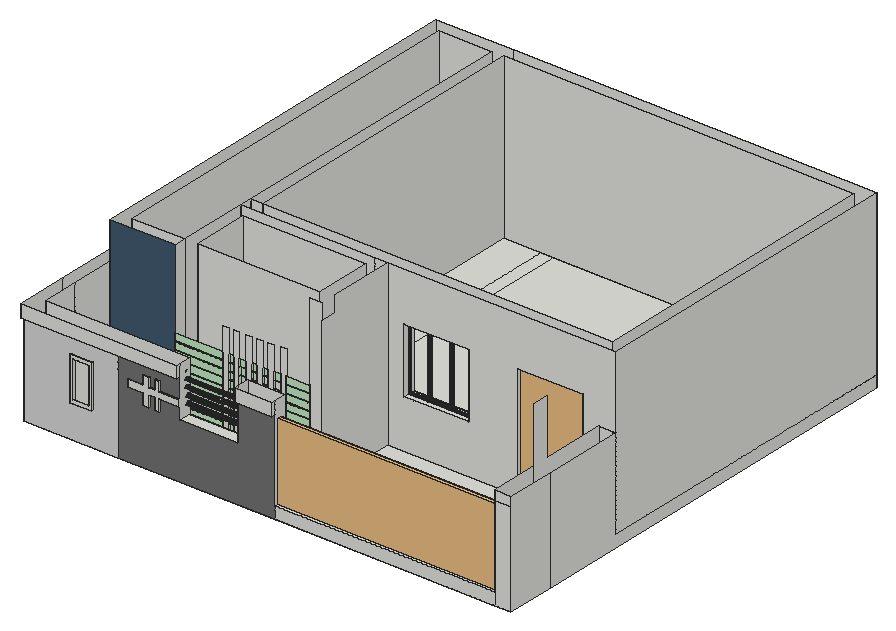
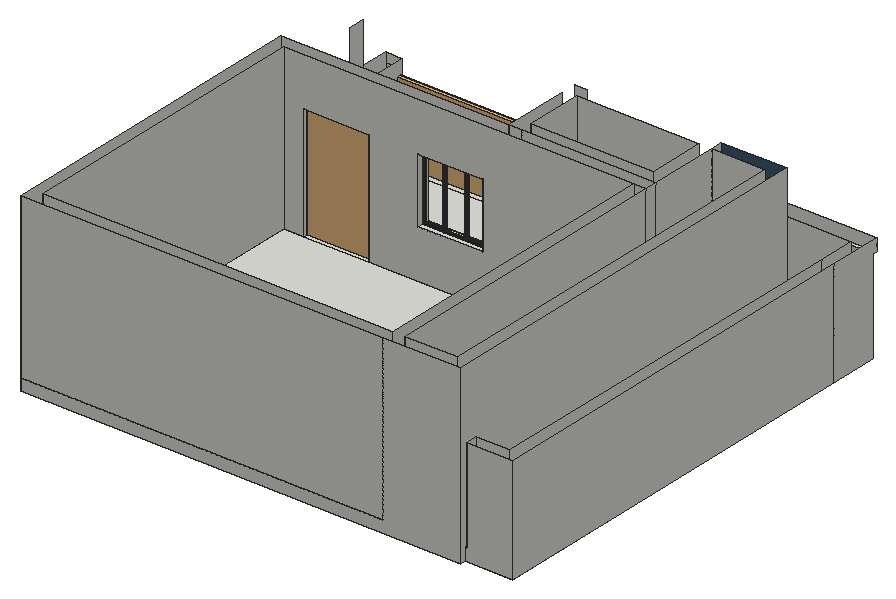
# SketchUp Ruby script. Lengths in inches.
U = 1.inch
M = Sketchup.active_model
def pt(a) = Geom::Point3d.new(a.map { |v| v * U })
def face(e, loops, mat)
  f = e.add_face(loops[0].map { |a| pt(a) })
  loops[1..].each { |l| e.add_face(l.map { |a| pt(a) }).erase! }
  f.material = f.back_material = mat if mat
  f
end
# faces: each face lists its corners as indices into pts; further lists are holes
def faces(e, pts, list, mat = nil) = list.each { |f| face(e, (f[0].is_a?(Array) ? f : [f]).map { |l| l.map { |i| pts[i] } }, mat) }
# xy, xz, yz: faces in a plane at the given z, y or x. An outline is a flat list of corners, or four numbers for a rectangle; further outlines are holes
def ring(l) = l.size == 4 ? [[l[0], l[1]], [l[2], l[1]], [l[2], l[3]], [l[0], l[3]]] : l.each_slice(2).to_a
def flat(e, list, mat, &to3) = list.each { |f| face(e, (f[0].is_a?(Array) ? f : [f]).map { |l| ring(l).map { |u, v| to3.(u, v) } }, mat) }
def xy(e, z, list, mat = nil) = flat(e, list, mat) { |x, y| [x, y, z] }
def xz(e, y, list, mat = nil) = flat(e, list, mat) { |x, z| [x, y, z] }
def yz(e, x, list, mat = nil) = flat(e, list, mat) { |y, z| [x, y, z] }
def lines(e, pts, list) = list.each { |a, b| e.add_line(pt(pts[a]), pt(pts[b])) }
# prism: a flat outline (further loops are holes) pulled along v
def prism(e, loops, v, mat = nil)
  f = face(e, loops, mat); d = Geom::Vector3d.new(v.map { |x| x * U })
  f.pushpull(f.normal.samedirection?(d) ? d.length : -d.length)
end
def box(e, o, s, mat = nil) = prism(e, [[o, [o[0] + s[0], o[1], o[2]], [o[0] + s[0], o[1] + s[1], o[2]], [o[0], o[1] + s[1], o[2]]]], [0, 0, s[2]], mat)
def at(x, y, z, deg = 0) = Geom::Transformation.translation(pt([x, y, z])) * Geom::Transformation.rotation(ORIGIN, Z_AXIS, deg.degrees)
def axes(o, x, y, z) = Geom::Transformation.new([*x, 0, *y, 0, *z, 0, *pt(o).to_a, 1])
def part(name) = M.definitions.add(name)
# library, detail: a bought-in or finely detailed component or shape, given as its bounding box
def library(name, o, s) = part(name).tap { |d| box(d.entities, o, s) }
def detail(e, o, s) = box(e.add_group.entities, o, s)
def put(e, d, t, mat = nil) = e.add_instance(d, t).tap { |i| i.material = mat if mat }
def group(e, t, mat = nil) = e.add_group.tap { |g| g.transformation = t; g.material = mat if mat }.entities
root = M.entities
M.materials.add("Wine2").color = [0, 0, 0]
M.materials["Wine2"].alpha = 0
M.materials.add("[0111_SlateGray]").color = [66, 89, 112]
M.materials.add("[0116_Lavender]").color = [195, 232, 195]
M.materials.add("[0128_White]").color = [214, 214, 214]
M.materials.add("[0130_Gainsboro]").color = [39, 45, 50]
M.materials.add("[0135_DarkGray]").color = [114, 114, 114]
c1 = library("porta 4",[0.2,-5.42,1.33],[46.55,4.72,83.21])
c2 = library("Louvered screen",[0,0,0],[122,4.25,84])
c3 = part("Framed glazing panel")
xy(c3.entities,0,[[0,-0.98,43.07,0],[0,0,43.07,1.4]],"[0130_Gainsboro]")
xy(c3.entities,0.3,[[0.3,-1.43,42.77,-0.98]],"[0130_Gainsboro]")
xy(c3.entities,2.95,[[2.95,-1.43,40.12,-0.63],[2.95,-0.63,40.12,0],[2.95,0,40.12,0.64],[2.95,0.64,40.12,1.4]],"[0130_Gainsboro]")
xy(c3.entities,3.54,[[3.54,-0.63,39.53,0],[3.54,0,39.53,0.64]],"[0130_Gainsboro]")
xy(c3.entities,111.8125,[[3.54,-0.63,39.53,0],[3.54,0,39.53,0.64]],"[0130_Gainsboro]")
xy(c3.entities,112.4,[[2.95,-1.43,40.12,-0.63],[2.95,-0.63,40.12,0],[2.95,0,40.12,0.64],[2.95,0.64,40.12,1.4]],"[0130_Gainsboro]")
xy(c3.entities,115.05,[[0.3,-1.43,42.77,-0.98]],"[0130_Gainsboro]")
xy(c3.entities,115.35,[[0,-0.98,43.07,0],[0,0,43.07,1.4]],"[0130_Gainsboro]")
xz(c3.entities,-1.43,[[[0.3,0.3,42.77,115.05],[2.95,2.95,40.12,112.4]]],"[0130_Gainsboro]")
xz(c3.entities,-0.98,[[[0,0,43.07,115.35],[0.3,0.3,42.77,115.05]]],"[0130_Gainsboro]")
xz(c3.entities,-0.63,[[[2.95,2.95,40.12,112.4],[3.54,3.54,39.53,111.8125]]],"[0130_Gainsboro]")
xz(c3.entities,0,[[3.54,3.54,39.53,111.8125]],"Wine2")
xz(c3.entities,0,[[[0,0,43.07,115.35],[2.95,2.95,40.12,112.4]],[[2.95,2.95,40.12,112.4],[3.54,3.54,39.53,111.8125]]],"[0130_Gainsboro]")
xz(c3.entities,0.64,[[[2.95,2.95,40.12,112.4],[3.54,3.54,39.53,111.8125]]],"[0130_Gainsboro]")
xz(c3.entities,1.4,[[[0,0,43.07,115.35],[2.95,2.95,40.12,112.4]]],"[0130_Gainsboro]")
yz(c3.entities,0,[[-0.98,0,0,115.35],[0,0,1.4,115.35]],"[0130_Gainsboro]")
yz(c3.entities,0.3,[[-1.43,0.3,-0.98,115.05]],"[0130_Gainsboro]")
yz(c3.entities,2.95,[[-1.43,2.95,-0.63,112.4],[-0.63,2.95,0,112.4],[0,2.95,0.64,112.4],[0.64,2.95,1.4,112.4]],"[0130_Gainsboro]")
yz(c3.entities,3.54,[[-0.63,3.54,0,111.8125],[0,3.54,0.64,111.8125]],"[0130_Gainsboro]")
yz(c3.entities,39.53,[[-0.63,3.54,0,111.8125],[0,3.54,0.64,111.8125]],"[0130_Gainsboro]")
yz(c3.entities,40.12,[[-1.43,2.95,-0.63,112.4],[-0.63,2.95,0,112.4],[0,2.95,0.64,112.4],[0.64,2.95,1.4,112.4]],"[0130_Gainsboro]")
yz(c3.entities,42.77,[[-1.43,0.3,-0.98,115.05]],"[0130_Gainsboro]")
yz(c3.entities,43.07,[[-0.98,0,0,115.35],[0,0,1.4,115.35]],"[0130_Gainsboro]")
c4 = part("Glazed window assembly")
put(c4.entities,c3,axes([90.57,1.43,0],[1.05148,0,0],[0,1,0],[0,0,1]))
put(c4.entities,c3,axes([0,1.43,0],[1.05148,0,0],[0,1,0],[0,0,1]))
put(c4.entities,c3,axes([45.29,1.43,0],[1.05148,0,0],[0,1,0],[0,0,1]))
xy(root,-9,[[0,3,359,39],[0,39,0,334.8,35,334.8,35,339,359,339,359,39]])
xy(root,0,[[185.01,3,347,12],[9,12,347,12,347,99,335,99,335,108,287,108,287,99,191,99,191,39,182,39,182,38.5,164.87,38.5,164.87,39,160.62,39,160.62,38.4375,156.37,38.4375,156.37,37.875,152.12,37.875,152.12,38.4375,148.37,38.4375,148.37,37.4375,144.12,37.4375,144.12,38.5,140.12,38.5,140.12,39,135.87,39,135.87,38.375,131.18,38.375,131.18,37.375,126.93,37.375,126.93,38.375,123.62,38.375,123.62,37.5625,119.37,37.5625,119.37,38.5,83,38.5,83,39,9,39],[126.93,37.375,131.18,39],[144.12,37.4375,148.37,39],[119.37,37.5625,123.62,39],
  [152.12,37.875,156.37,39],[123.62,38.375,126.93,39],[131.18,38.375,135.87,39],[148.37,38.4375,152.12,39],[156.37,38.4375,160.62,39],
  [83,38.5,119.37,39],[140.12,38.5,144.12,39],[164.87,38.5,182,39],[9,39,35,39,35,334.8,34,334.8,34,325.8,9,325.8],[[83,39,191,99],[92,48,182,90]],
  [44,48,83,330],[92,48,182,90],[83,99,287,108],[350,99,359,99,359,339,92,339,92,330,350,330],[335,99,350,108],
  [92,108,119,330],[119,108,128,330],[128,108,350,330]])
xy(root,5,[[123.62,38.375,126.93,39],[131.18,38.375,135.87,39],[148.37,38.4375,152.12,39],[156.37,38.4375,160.62,39],[83,38.5,119.37,39],
  [140.12,38.5,144.12,39],[164.87,38.5,182,39]])
xy(root,5.75,[[123.62,38.375,126.93,39],[131.18,38.375,135.87,39],[148.37,38.4375,152.12,39],[156.37,38.4375,160.62,39],[83,38.5,119.37,39],
  [140.12,38.5,144.12,39],[164.87,38.5,182,39]])
xy(root,10.75,[[123.62,38.375,126.93,39],[131.18,38.375,135.87,39],[148.37,38.4375,152.12,39],[156.37,38.4375,160.62,39],[83,38.5,119.37,39],
  [140.12,38.5,144.12,39],[164.87,38.5,182,39]])
xy(root,11.5,[[148.37,38.4375,152.12,39],[156.37,38.4375,160.62,39],[83,38.5,119.37,39],[123.62,38.5,126.93,39],[131.18,38.5,135.87,39],
  [140.12,38.5,144.12,39],[164.87,38.5,182,39]])
xy(root,15.77,[[35.15,2,50.69,3]])
xy(root,16.5,[[148.37,38.4375,152.12,39],[156.37,38.4375,160.62,39],[83,38.5,119.37,39],[123.62,38.5,126.93,39],[131.18,38.5,135.87,39],
  [140.12,38.5,144.12,39],[164.87,38.5,182,39]])
xy(root,17.25,[[148.37,38.4375,152.12,39],[83,38.5,119.37,39],[123.62,38.5,126.93,39],[131.18,38.5,135.87,39],[140.12,38.5,144.12,39],
  [156.37,38.5,160.62,39],[164.87,38.5,182,39]])
xy(root,17.98,[[37.36,2,48.48,3]])
xy(root,22.25,[[148.37,38.4375,152.12,39],[83,38.5,119.37,39],[123.62,38.5,126.93,39],[131.18,38.5,135.87,39],[140.12,38.5,144.12,39],
  [156.37,38.5,160.62,39],[164.87,38.5,182,39]])
xy(root,23,[[83,38.5,119.37,39],[123.62,38.5,126.93,39],[131.18,38.5,135.87,39],[140.12,38.5,144.12,39],[148.37,38.5,152.12,39],
  [156.37,38.5,160.62,39],[164.87,38.5,182,39]])
xy(root,28,[[83,38.5,119.37,39],[123.62,38.5,126.93,39],[131.18,38.5,135.87,39],[140.12,38.5,144.12,39],[148.37,38.5,152.12,39],
  [156.37,38.5,160.62,39],[164.87,38.5,182,39]])
xy(root,28.75,[[135.87,37.4375,140.12,39],[83,38.5,119.37,39],[123.62,38.5,126.93,39],[131.18,38.5,135.87,39],[140.12,38.5,144.12,39],
  [148.37,38.5,152.12,39],[156.37,38.5,160.62,39],[164.87,38.5,182,39]])
xy(root,31.67,[[115.21,3,157.75,12]])
xy(root,32.31,[[97.17,2,100.67,3]])
xy(root,32.63,[[88.58,2,92.7,3]])
xy(root,33.75,[[83,38.5,119.37,39],[123.62,38.5,126.93,39],[131.18,38.5,135.87,39],[140.12,38.5,144.12,39],[148.37,38.5,152.12,39],
  [156.37,38.5,160.62,39],[164.87,38.5,182,39]])
xy(root,34.5,[[83,38.5,119.37,39],[123.62,38.5,126.93,39],[131.18,38.5,135.87,39],[140.12,38.5,144.12,39],[148.37,38.5,152.12,39],
  [156.37,38.5,160.62,39],[164.87,38.5,182,39]])
xy(root,36,[[203,99,251,108]])
xy(root,39.5,[[83,38.5,119.37,39],[123.62,38.5,126.93,39],[131.18,38.5,135.87,39],[140.12,38.5,144.12,39],[148.37,38.5,152.12,39],
  [156.37,38.5,160.62,39],[164.87,38.5,182,39]])
xy(root,40.25,[[155.87,37.875,156.37,38.5],[83,38.5,119.37,39],[123.62,38.5,126.93,39],[131.18,38.5,135.87,39],[140.12,38.5,144.12,39],
  [148.37,38.5,152.12,39],[156.37,38.5,160.62,39],[164.87,38.5,182,39]])
xy(root,40.9,[[77.4,2,88.58,3],[92.7,2,97.17,3],[100.67,2,115.21,3]])
xy(root,45.25,[[155.87,37.875,156.37,38.5],[83,38.5,119.37,39],[123.62,38.5,126.93,39],[131.18,38.5,135.87,39],[140.12,38.5,144.12,39],
  [148.37,38.5,152.12,39],[156.37,38.5,160.62,39],[164.87,38.5,182,39]])
xy(root,45.36,[[37.36,2,48.48,3]])
xy(root,45.83,[[77.4,2,88.58,3],[92.7,2,97.17,3],[100.67,2,115.21,3]])
xy(root,46,[[83,38.5,119.37,39],[131.18,38.5,135.87,39],[140.12,38.5,144.12,39],[148.37,38.5,152.12,39],[156.37,38.5,160.62,39],
  [164.87,38.5,182,39],[123.62,38.625,126.93,39]])
xy(root,47.5625,[[35.15,2,50.69,3]])
xy(root,51,[[83,38.5,119.37,39],[131.18,38.5,135.87,39],[140.12,38.5,144.12,39],[148.37,38.5,152.12,39],[156.37,38.5,160.62,39],
  [164.87,38.5,182,39],[123.62,38.625,126.93,39]])
xy(root,51.75,[[83,38.5,119.37,39],[131.18,38.5,135.87,39],[140.12,38.5,144.12,39],[148.37,38.5,152.12,39],[156.37,38.5,160.62,39],
  [164.87,38.5,182,39],[123.62,38.625,126.93,39]])
xy(root,52.38,[[88.58,2,92.7,3]])
xy(root,52.43,[[97.17,2,100.67,3]])
xy(root,56.75,[[83,38.5,119.37,39],[131.18,38.5,135.87,39],[140.12,38.5,144.12,39],[148.37,38.5,152.12,39],[156.37,38.5,160.62,39],
  [164.87,38.5,182,39],[123.62,38.625,126.93,39]])
xy(root,57.5,[[131.18,38.4375,135.87,39],[83,38.5,119.37,39],[140.12,38.5,144.12,39],[148.37,38.5,152.12,39],[156.37,38.5,160.62,39],
  [164.87,38.5,182,39],[123.62,38.625,126.93,39]])
xy(root,60,[[0,0,115.21,3],[157.75,0,185.01,3]])
xz(root,0,[[0,60,115.21,69],[157.75,60,185.01,69]])
xz(root,2,[[[35.15,15.77,50.69,47.5625],[37.36,17.98,48.48,45.36]],[97.17,32.31,100.67,32.31,100.67,40.9,115.21,40.9,115.21,45.83,100.67,45.83,100.67,52.43,97.17,52.43,97.17,45.83,92.7,45.83,92.7,52.38,88.58,52.38,88.58,45.83,77.4,45.83,77.4,40.9,88.58,40.9,88.58,32.63,92.7,32.63,92.7,40.9,97.17,40.9]])
xz(root,3,[[185.01,-9,347,0],[347,-9,359,60],[37.36,17.98,48.48,45.36],[347,60,359,67]])
xz(root,3,[[[0,-9,69.1875,60],[35.15,15.77,50.69,47.5625]]],"[0128_White]")
xz(root,3,[[69.1875,-9,185.01,-9,185.01,60,157.75,60,157.75,31.67,115.21,31.67,115.21,40.9,100.67,40.9,100.67,32.31,97.17,32.31,97.17,40.9,92.7,40.9,92.7,32.63,88.58,32.63,88.58,40.9,77.4,40.9,77.4,45.83,88.58,45.83,88.58,52.38,92.7,52.38,92.7,45.83,97.17,45.83,97.17,52.43,100.67,52.43,100.67,45.83,115.21,45.83,115.21,60,69.1875,60]],"[0135_DarkGray]")
xz(root,12,[[9,0,9,69,115.21,69,115.21,31.67,157.75,31.67,157.75,69,185.01,69,185.01,0]])
xz(root,37.375,[[126.93,0,131.18,80.25]])
xz(root,37.4375,[[144.12,0,148.37,80.25],[135.87,28.75,140.12,80.25]])
xz(root,37.5625,[[119.37,0,123.62,80.25]])
xz(root,37.875,[[152.12,0,156.37,0,156.37,40.25,155.87,40.25,155.87,45.25,156.37,45.25,156.37,80.25,152.12,80.25]])
xz(root,38.375,[[123.62,0,126.93,5],[131.18,0,135.87,5],[123.62,5.75,126.93,10.75],[131.18,5.75,135.87,10.75]],"[0116_Lavender]")
xz(root,38.4375,[[148.37,0,152.12,5],[156.37,0,160.62,5],[148.37,5.75,152.12,10.75],[156.37,5.75,160.62,10.75],[148.37,11.5,152.12,16.5],
  [156.37,11.5,160.62,16.5],[148.37,17.25,152.12,22.25],[131.18,57.5,135.87,62.5]],"[0116_Lavender]")
xz(root,38.5,[[140.12,0,144.12,5],[155.87,40.25,160.62,45.25],[148.37,46,152.12,51],[156.37,46,160.62,51],[148.37,51.75,152.12,56.75],
  [156.37,51.75,160.62,56.75]])
xz(root,38.5,[[83,0,119.37,5],[164.87,0,182,5],[83,5.75,119.37,10.75],[140.12,5.75,144.12,10.75],[164.87,5.75,182,10.75],
  [83,11.5,119.37,16.5],[123.62,11.5,126.93,16.5],[131.18,11.5,135.87,16.5],[140.12,11.5,144.12,16.5],[164.87,11.5,182,16.5],
  [83,17.25,119.37,22.25],[123.62,17.25,126.93,22.25],[131.18,17.25,135.87,22.25],[140.12,17.25,144.12,22.25],[156.37,17.25,160.62,22.25],
  [164.87,17.25,182,22.25],[83,23,119.37,28],[123.62,23,126.93,28],[131.18,23,135.87,28],[140.12,23,144.12,28],
  [148.37,23,152.12,28],[156.37,23,160.62,28],[164.87,23,182,28],[83,28.75,119.37,33.75],[123.62,28.75,126.93,33.75],
  [131.18,28.75,135.87,33.75],[140.12,28.75,144.12,33.75],[148.37,28.75,152.12,33.75],[156.37,28.75,160.62,33.75],[164.87,28.75,182,33.75],
  [83,34.5,119.37,39.5],[123.62,34.5,126.93,39.5],[131.18,34.5,135.87,39.5],[140.12,34.5,144.12,39.5],[148.37,34.5,152.12,39.5],
  [156.37,34.5,160.62,39.5],[164.87,34.5,182,39.5],[83,40.25,119.37,45.25],[123.62,40.25,126.93,45.25],[131.18,40.25,135.87,45.25],
  [140.12,40.25,144.12,45.25],[148.37,40.25,152.12,45.25],[164.87,40.25,182,45.25],[83,46,119.37,51],[131.18,46,135.87,51],
  [140.12,46,144.12,51],[164.87,46,182,51],[83,51.75,119.37,56.75],[131.18,51.75,135.87,56.75],[140.12,51.75,144.12,56.75],
  [164.87,51.75,182,56.75],[83,57.5,119.37,62.5],[140.12,57.5,144.12,62.5],[148.37,57.5,152.12,62.5],[156.37,57.5,160.62,62.5],
  [164.87,57.5,182,62.5]],"[0116_Lavender]")
xz(root,38.625,[[123.62,46,126.93,51],[123.62,51.75,126.93,56.75],[123.62,57.5,126.93,62.5]],"[0116_Lavender]")
xz(root,39,[[135.87,0,140.12,28.75],[160.62,0,164.87,28],[182,0,191,120],[83,5,119.37,5.75],[123.62,5,126.93,5.75],
  [131.18,5,135.87,5.75],[140.12,5,144.12,5.75],[148.37,5,152.12,5.75],[156.37,5,160.62,5.75],[164.87,5,182,5.75],
  [83,10.75,119.37,11.5],[123.62,10.75,126.93,11.5],[131.18,10.75,135.87,11.5],[140.12,10.75,144.12,11.5],[148.37,10.75,152.12,11.5],
  [156.37,10.75,160.62,11.5],[164.87,10.75,182,11.5],[83,16.5,119.37,17.25],[123.62,16.5,126.93,17.25],[131.18,16.5,135.87,17.25],
  [140.12,16.5,144.12,17.25],[148.37,16.5,152.12,17.25],[156.37,16.5,160.62,17.25],[164.87,16.5,182,17.25],[83,22.25,119.37,23],
  [123.62,22.25,126.93,23],[131.18,22.25,135.87,23],[140.12,22.25,144.12,23],[148.37,22.25,152.12,23],[156.37,22.25,160.62,23],
  [164.87,22.25,182,23],[83,28,119.37,28.75],[123.62,28,126.93,28.75],[131.18,28,135.87,28.75],[140.12,28,144.12,28.75],
  [148.37,28,152.12,28.75],[156.37,28,160.62,28.75],[160.62,28,164.87,80.25],[164.87,28,182,28.75],[83,33.75,119.37,34.5],
  [123.62,33.75,126.93,34.5],[131.18,33.75,135.87,34.5],[140.12,33.75,144.12,34.5],[148.37,33.75,152.12,34.5],[156.37,33.75,160.62,34.5],
  [164.87,33.75,182,34.5],[83,39.5,119.37,40.25],[123.62,39.5,126.93,40.25],[131.18,39.5,135.87,40.25],[140.12,39.5,144.12,40.25],
  [148.37,39.5,152.12,40.25],[156.37,39.5,160.62,40.25],[164.87,39.5,182,40.25],[83,45.25,119.37,46],[123.62,45.25,126.93,46],
  [131.18,45.25,135.87,46],[140.12,45.25,144.12,46],[148.37,45.25,152.12,46],[156.37,45.25,160.62,46],[164.87,45.25,182,46],
  [83,51,119.37,51.75],[123.62,51,126.93,51.75],[131.18,51,135.87,51.75],[140.12,51,144.12,51.75],[148.37,51,152.12,51.75],
  [156.37,51,160.62,51.75],[164.87,51,182,51.75],[83,56.75,119.37,57.5],[123.62,56.75,126.93,57.5],[131.18,56.75,135.87,57.5],
  [140.12,56.75,144.12,57.5],[148.37,56.75,152.12,57.5],[156.37,56.75,160.62,57.5],[164.87,56.75,182,57.5]])
xz(root,39,[[35,0,83,120]],"[0111_SlateGray]")
xz(root,48,[[44,0,83,120],[92,0,182,120]])
xz(root,90,[[92,0,182,120]])
xz(root,99,[[83,0,182,120],[182,0,191,120],[[191,0,287,0,287,84,335,84,335,0,347,0,347,67,359,67,359,120,191,120],[203,36,251,84]]])
xz(root,108,[[83,0,92,120],[[92,0,92,120,350,120,350,0,335,0,335,84,287,84,287,0],[203,36,251,84]]])
xz(root,325.8,[[9,0,34,69]])
xz(root,330,[[44,0,83,120],[92,0,350,120]])
xz(root,334.8,[[0,-9,0,69,34,69,34,0,35,0,35,-9]])
xz(root,339,[[35,-9,35,120,92,120,92,0,359,0,359,-9],[92,0,359,120]])
yz(root,0,[[3,-9,3,60,0,60,0,69,39,69,39,-9],[39,-9,334.8,69]])
yz(root,9,[[12,0,39,69],[39,0,325.8,69]])
yz(root,34,[[325.8,0,334.8,69]])
yz(root,35,[[334.8,-9,334.8,0,39,0,39,120,339,120,339,-9]])
yz(root,35.15,[[2,15.77,3,47.5625]])
yz(root,37.36,[[2,17.98,3,45.36]])
yz(root,44,[[48,0,330,120]])
yz(root,48.48,[[2,17.98,3,45.36]])
yz(root,50.69,[[2,15.77,3,47.5625]])
yz(root,77.4,[[2,40.9,3,45.83]])
yz(root,83,[[38.5,0,39,5],[39,0,48,120],[48,0,99,120],[99,0,108,120],[108,0,330,120],
  [38.5,5.75,39,10.75],[38.5,11.5,39,16.5],[38.5,17.25,39,22.25],[38.5,23,39,28],[38.5,28.75,39,33.75],
  [38.5,34.5,39,39.5],[38.5,40.25,39,45.25],[38.5,46,39,51],[38.5,51.75,39,56.75],[38.5,57.5,39,62.5]])
yz(root,88.58,[[2,32.63,3,40.9],[2,45.83,3,52.38]])
yz(root,92,[[48,0,90,120],[108,0,330,120]])
yz(root,92.7,[[2,32.63,3,40.9],[2,45.83,3,52.38]])
yz(root,97.17,[[2,32.31,3,40.9],[2,45.83,3,52.43]])
yz(root,100.67,[[2,32.31,3,40.9],[2,45.83,3,52.43]])
yz(root,115.21,[[[3,31.67,12,31.67,12,69,3,69,3,45.83,2,45.83,2,40.9,3,40.9],[9.375,44.125,9.05,44.17,8.75,44.29,8.49,44.49,8.29,44.75,8.17,45.05,8.125,45.375,8.17,45.7,8.29,46,8.49,46.26,8.75,46.46,9.05,46.58,9.375,46.625,9.7,46.58,10,46.46,10.26,46.26,10.46,46,10.58,45.7,10.625,45.375,10.58,45.05,10.46,44.75,10.26,44.49,10,44.29,9.7,44.17],[9.375,38.875,9.05,38.92,8.75,39.04,8.49,39.24,8.29,39.5,8.17,39.8,8.125,40.125,8.17,40.45,8.29,40.75,8.49,41.01,8.75,41.21,9.05,41.33,9.375,41.375,9.7,41.33,10,41.21,10.26,41.01,10.46,40.75,10.58,40.45,10.625,40.125,10.58,39.8,10.46,39.5,10.26,39.24,10,39.04,9.7,38.92],[8.625,50.42,8.33,50.46,8.0625,50.57,7.83,50.75,7.65,50.99,7.54,51.26,7.5,51.55,7.54,51.84,7.65,52.11,7.83,52.34,8.0625,52.52,8.33,52.63,8.625,52.67,8.92,52.63,9.1875,52.52,9.42,52.34,9.6,52.11,9.71,51.84,9.75,51.55,9.71,51.26,9.6,50.99,9.42,50.75,9.1875,50.57,8.92,50.46],[8.625,60.67,8.33,60.71,8.0625,60.82,7.83,61,7.65,61.24,7.54,61.51,7.5,61.8,7.54,62.09,7.65,62.36,7.83,62.59,8.0625,62.77,8.33,62.88,8.625,62.92,8.92,62.88,9.1875,62.77,9.42,62.59,9.6,62.36,9.71,62.09,9.75,61.8,9.71,61.51,9.6,61.24,9.42,61,9.1875,60.82,8.92,60.71],[8.625,55.8,8.33,55.84,8.0625,55.95,7.83,56.13,7.65,56.36,7.54,56.63,7.5,56.92,7.54,57.21,7.65,57.49,7.83,57.72,8.0625,57.9,8.33,58.01,8.625,58.05,8.92,58.01,9.1875,57.9,9.42,57.72,9.6,57.49,9.71,57.21,9.75,56.92,9.71,56.63,9.6,56.36,9.42,56.13,9.1875,55.95,8.92,55.84]],[0,60,3,69]])
yz(root,119.37,[[37.5625,0,38.5,5],[37.5625,5,39,5.75],[37.5625,5.75,38.5,10.75],[37.5625,10.75,39,11.5],[37.5625,11.5,38.5,16.5],
  [37.5625,16.5,39,17.25],[37.5625,17.25,38.5,22.25],[37.5625,22.25,39,23],[37.5625,23,38.5,28],[37.5625,28,39,28.75],
  [37.5625,28.75,38.5,33.75],[37.5625,33.75,39,34.5],[37.5625,34.5,38.5,39.5],[37.5625,39.5,39,40.25],[37.5625,40.25,38.5,45.25],
  [37.5625,45.25,39,46],[37.5625,46,38.5,51],[37.5625,51,39,51.75],[37.5625,51.75,38.5,56.75],[37.5625,56.75,39,57.5],
  [37.5625,57.5,38.5,62.5]])
yz(root,123.62,[[37.5625,0,38.375,5],[37.5625,5,39,5.75],[37.5625,5.75,38.375,10.75],[37.5625,10.75,39,11.5],[37.5625,11.5,38.5,16.5],
  [37.5625,16.5,39,17.25],[37.5625,17.25,38.5,22.25],[37.5625,22.25,39,23],[37.5625,23,38.5,28],[37.5625,28,39,28.75],
  [37.5625,28.75,38.5,33.75],[37.5625,33.75,39,34.5],[37.5625,34.5,38.5,39.5],[37.5625,39.5,39,40.25],[37.5625,40.25,38.5,45.25],
  [37.5625,45.25,39,46],[37.5625,46,38.625,51],[37.5625,51,39,51.75],[37.5625,51.75,38.625,56.75],[37.5625,56.75,39,57.5],
  [37.5625,57.5,38.625,62.5]])
yz(root,126.93,[[37.375,0,38.375,5],[37.375,5,39,5.75],[37.375,5.75,38.375,10.75],[37.375,10.75,39,11.5],[37.375,11.5,38.5,16.5],
  [37.375,16.5,39,17.25],[37.375,17.25,38.5,22.25],[37.375,22.25,39,23],[37.375,23,38.5,28],[37.375,28,39,28.75],
  [37.375,28.75,38.5,33.75],[37.375,33.75,39,34.5],[37.375,34.5,38.5,39.5],[37.375,39.5,39,40.25],[37.375,40.25,38.5,45.25],
  [37.375,45.25,39,46],[37.375,46,38.625,51],[37.375,51,39,51.75],[37.375,51.75,38.625,56.75],[37.375,56.75,39,57.5],
  [37.375,57.5,38.625,62.5]])
yz(root,131.18,[[37.375,0,38.375,5],[37.375,5,39,5.75],[37.375,5.75,38.375,10.75],[37.375,10.75,39,11.5],[37.375,11.5,38.5,16.5],
  [37.375,16.5,39,17.25],[37.375,17.25,38.5,22.25],[37.375,22.25,39,23],[37.375,23,38.5,28],[37.375,28,39,28.75],
  [37.375,28.75,38.5,33.75],[37.375,33.75,39,34.5],[37.375,34.5,38.5,39.5],[37.375,39.5,39,40.25],[37.375,40.25,38.5,45.25],
  [37.375,45.25,39,46],[37.375,46,38.5,51],[37.375,51,39,51.75],[37.375,51.75,38.5,56.75],[37.375,56.75,39,57.5],
  [37.375,57.5,38.4375,62.5]])
yz(root,135.87,[[38.375,0,39,5],[38.375,5.75,39,10.75],[38.5,11.5,39,16.5],[38.5,17.25,39,22.25],[38.5,23,39,28],
  [37.4375,28.75,38.5,33.75],[37.4375,33.75,39,34.5],[37.4375,34.5,38.5,39.5],[37.4375,39.5,39,40.25],[37.4375,40.25,38.5,45.25],
  [37.4375,45.25,39,46],[37.4375,46,38.5,51],[37.4375,51,39,51.75],[37.4375,51.75,38.5,56.75],[37.4375,56.75,39,57.5],
  [37.4375,57.5,38.4375,62.5]])
yz(root,140.12,[[38.5,0,39,5],[38.5,5.75,39,10.75],[38.5,11.5,39,16.5],[38.5,17.25,39,22.25],[38.5,23,39,28],
  [37.4375,28.75,38.5,33.75],[37.4375,33.75,39,34.5],[37.4375,34.5,38.5,39.5],[37.4375,39.5,39,40.25],[37.4375,40.25,38.5,45.25],
  [37.4375,45.25,39,46],[37.4375,46,38.5,51],[37.4375,51,39,51.75],[37.4375,51.75,38.5,56.75],[37.4375,56.75,39,57.5],
  [37.4375,57.5,38.5,62.5]])
yz(root,144.12,[[37.4375,0,38.5,5],[37.4375,5,39,5.75],[37.4375,5.75,38.5,10.75],[37.4375,10.75,39,11.5],[37.4375,11.5,38.5,16.5],
  [37.4375,16.5,39,17.25],[37.4375,17.25,38.5,22.25],[37.4375,22.25,39,23],[37.4375,23,38.5,28],[37.4375,28,39,28.75],
  [37.4375,28.75,38.5,33.75],[37.4375,33.75,39,34.5],[37.4375,34.5,38.5,39.5],[37.4375,39.5,39,40.25],[37.4375,40.25,38.5,45.25],
  [37.4375,45.25,39,46],[37.4375,46,38.5,51],[37.4375,51,39,51.75],[37.4375,51.75,38.5,56.75],[37.4375,56.75,39,57.5],
  [37.4375,57.5,38.5,62.5]])
yz(root,148.37,[[37.4375,0,38.4375,5],[37.4375,5,39,5.75],[37.4375,5.75,38.4375,10.75],[37.4375,10.75,39,11.5],[37.4375,11.5,38.4375,16.5],
  [37.4375,16.5,39,17.25],[37.4375,17.25,38.4375,22.25],[37.4375,22.25,39,23],[37.4375,23,38.5,28],[37.4375,28,39,28.75],
  [37.4375,28.75,38.5,33.75],[37.4375,33.75,39,34.5],[37.4375,34.5,38.5,39.5],[37.4375,39.5,39,40.25],[37.4375,40.25,38.5,45.25],
  [37.4375,45.25,39,46],[37.4375,46,38.5,51],[37.4375,51,39,51.75],[37.4375,51.75,38.5,56.75],[37.4375,56.75,39,57.5],
  [37.4375,57.5,38.5,62.5]])
yz(root,152.12,[[37.875,0,38.4375,5],[37.875,5,39,5.75],[37.875,5.75,38.4375,10.75],[37.875,10.75,39,11.5],[37.875,11.5,38.4375,16.5],
  [37.875,16.5,39,17.25],[37.875,17.25,38.4375,22.25],[37.875,22.25,39,23],[37.875,23,38.5,28],[37.875,28,39,28.75],
  [37.875,28.75,38.5,33.75],[37.875,33.75,39,34.5],[37.875,34.5,38.5,39.5],[37.875,39.5,39,40.25],[37.875,40.25,38.5,45.25],
  [37.875,45.25,39,46],[37.875,46,38.5,51],[37.875,51,39,51.75],[37.875,51.75,38.5,56.75],[37.875,56.75,39,57.5],
  [37.875,57.5,38.5,62.5]])
yz(root,155.87,[[37.875,40.25,38.5,45.25]])
yz(root,156.37,[[37.875,0,38.4375,5],[37.875,5,39,5.75],[37.875,5.75,38.4375,10.75],[37.875,10.75,39,11.5],[37.875,11.5,38.4375,16.5],
  [37.875,16.5,39,17.25],[37.875,17.25,38.5,22.25],[37.875,22.25,39,23],[37.875,23,38.5,28],[37.875,28,39,28.75],
  [37.875,28.75,38.5,33.75],[37.875,33.75,39,34.5],[37.875,34.5,38.5,39.5],[37.875,39.5,39,40.25],[37.875,45.25,39,46],
  [37.875,46,38.5,51],[37.875,51,39,51.75],[37.875,51.75,38.5,56.75],[37.875,56.75,39,57.5],[37.875,57.5,38.5,62.5]])
yz(root,157.59,[[9.375,38.875,9.7,38.92,10,39.04,10.26,39.24,10.46,39.5,10.58,39.8,10.625,40.125,10.58,40.45,10.46,40.75,10.26,41.01,10,41.21,9.7,41.33,9.375,41.375,9.05,41.33,8.75,41.21,8.49,41.01,8.29,40.75,8.17,40.45,8.125,40.125,8.17,39.8,8.29,39.5,8.49,39.24,8.75,39.04,9.05,38.92]])
yz(root,157.75,[[[3,31.67,12,69],[9.375,44.125,9.7,44.17,10,44.29,10.26,44.49,10.46,44.75,10.58,45.05,10.625,45.375,10.58,45.7,10.46,46,10.26,46.26,10,46.46,9.7,46.58,9.375,46.625,9.05,46.58,8.75,46.46,8.49,46.26,8.29,46,8.17,45.7,8.125,45.375,8.17,45.05,8.29,44.75,8.49,44.49,8.75,44.29,9.05,44.17],[8.625,50.42,8.92,50.46,9.1875,50.57,9.42,50.75,9.6,50.99,9.71,51.26,9.75,51.55,9.71,51.84,9.6,52.11,9.42,52.34,9.1875,52.52,8.92,52.63,8.625,52.67,8.33,52.63,8.0625,52.52,7.83,52.34,7.65,52.11,7.54,51.84,7.5,51.55,7.54,51.26,7.65,50.99,7.83,50.75,8.0625,50.57,8.33,50.46]],[0,60,3,69]])
yz(root,157.9,[[8.625,55.8,8.92,55.84,9.1875,55.95,9.42,56.13,9.6,56.36,9.71,56.63,9.75,56.92,9.71,57.21,9.6,57.49,9.42,57.72,9.1875,57.9,8.92,58.01,8.625,58.05,8.33,58.01,8.0625,57.9,7.83,57.72,7.65,57.49,7.54,57.21,7.5,56.92,7.54,56.63,7.65,56.36,7.83,56.13,8.0625,55.95,8.33,55.84]])
yz(root,160.62,[[38.4375,0,39,5],[38.4375,5.75,39,10.75],[38.4375,11.5,39,16.5],[38.5,17.25,39,22.25],[38.5,23,39,28],
  [38.5,28.75,39,33.75],[38.5,34.5,39,39.5],[38.5,40.25,39,45.25],[38.5,46,39,51],[38.5,51.75,39,56.75],
  [38.5,57.5,39,62.5]])
yz(root,164.87,[[38.5,0,39,5],[38.5,5.75,39,10.75],[38.5,11.5,39,16.5],[38.5,17.25,39,22.25],[38.5,23,39,28],
  [38.5,28.75,39,33.75],[38.5,34.5,39,39.5],[38.5,40.25,39,45.25],[38.5,46,39,51],[38.5,51.75,39,56.75],
  [38.5,57.5,39,62.5]])
yz(root,182,[[38.5,0,39,5],[48,0,90,120],[38.5,5.75,39,10.75],[38.5,11.5,39,16.5],[38.5,17.25,39,22.25],
  [38.5,23,39,28],[38.5,28.75,39,33.75],[38.5,34.5,39,39.5],[38.5,40.25,39,45.25],[38.5,46,39,51],
  [38.5,51.75,39,56.75],[38.5,57.5,39,62.5]])
yz(root,185.01,[[3,0,12,69],[0,60,3,69]])
yz(root,191,[[39,0,99,0,99,120,51,120,51,108,39,108]])
yz(root,203,[[99,36,108,84]])
yz(root,251,[[99,36,108,84]])
yz(root,287,[[99,0,108,84]])
yz(root,335,[[99,0,108,84]])
yz(root,347,[[3,0,39,67],[39,0,39,108,51,108,51,67,99,67,99,0]])
yz(root,350,[[108,0,330,120]])
yz(root,359,[[3,-9,39,67],[39,-9,339,-9,339,0,99,0,99,67,39,67],[99,0,339,120]])
p = [[115.21,8.75,39.04],[115.21,9.05,38.92],[157.59,9.05,38.92],[157.59,8.75,39.04],[115.21,9.375,38.875],[157.59,9.375,38.875],
  [115.21,9.7,38.92],[157.59,9.7,38.92],[115.21,10,39.04],[157.59,10,39.04],[115.21,8.49,39.24],[157.59,8.49,39.24],
  [115.21,10.26,39.24],[157.59,10.26,39.24],[115.21,8.29,39.5],[157.59,8.29,39.5],[115.21,10.46,39.5],[157.59,10.46,39.5],
  [115.21,8.17,39.8],[157.59,8.17,39.8],[115.21,10.58,39.8],[157.59,10.58,39.8],[115.21,8.125,40.125],[157.59,8.125,40.125],
  [115.21,10.625,40.125],[157.59,10.625,40.125],[115.21,8.17,40.45],[157.59,8.17,40.45],[115.21,10.58,40.45],[157.59,10.58,40.45],
  [115.21,8.29,40.75],[157.59,8.29,40.75],[115.21,10.46,40.75],[157.59,10.46,40.75],[115.21,8.49,41.01],[157.59,8.49,41.01],
  [115.21,10.26,41.01],[157.59,10.26,41.01],[115.21,8.75,41.21],[157.59,8.75,41.21],[115.21,10,41.21],[157.59,10,41.21],
  [115.21,9.05,41.33],[157.59,9.05,41.33],[115.21,9.7,41.33],[157.59,9.7,41.33],[115.21,9.375,41.375],[157.59,9.375,41.375],
  [115.21,9.05,44.17],[115.21,9.375,44.125],[157.75,9.375,44.125],[157.75,9.05,44.17],[115.21,9.7,44.17],[157.75,9.7,44.17],
  [115.21,8.75,44.29],[157.75,8.75,44.29],[115.21,10,44.29],[157.75,10,44.29],[115.21,8.49,44.49],[157.75,8.49,44.49],
  [115.21,10.26,44.49],[157.75,10.26,44.49],[115.21,8.29,44.75],[157.75,8.29,44.75],[115.21,10.46,44.75],[157.75,10.46,44.75],
  [115.21,8.17,45.05],[157.75,8.17,45.05],[115.21,10.58,45.05],[157.75,10.58,45.05],[115.21,8.125,45.375],[157.75,8.125,45.375],
  [115.21,10.625,45.375],[157.75,10.625,45.375],[115.21,8.17,45.7],[157.75,8.17,45.7],[115.21,10.58,45.7],[157.75,10.58,45.7],
  [115.21,8.29,46],[157.75,8.29,46],[115.21,10.46,46],[157.75,10.46,46],[115.21,8.49,46.26],[157.75,8.49,46.26],
  [115.21,10.26,46.26],[157.75,10.26,46.26],[115.21,8.75,46.46],[157.75,8.75,46.46],[115.21,10,46.46],[157.75,10,46.46],
  [115.21,9.05,46.58],[157.75,9.05,46.58],[115.21,9.7,46.58],[157.75,9.7,46.58],[115.21,9.375,46.625],[157.75,9.375,46.625],
  [115.21,8.33,50.46],[115.21,8.625,50.42],[157.75,8.625,50.42],[157.75,8.33,50.46],[115.21,8.92,50.46],[157.75,8.92,50.46],
  [115.21,8.0625,50.57],[157.75,8.0625,50.57],[115.21,9.1875,50.57],[157.75,9.1875,50.57],[115.21,7.83,50.75],[157.75,7.83,50.75],
  [115.21,9.42,50.75],[157.75,9.42,50.75],[115.21,7.65,50.99],[157.75,7.65,50.99],[115.21,9.6,50.99],[157.75,9.6,50.99],
  [115.21,7.54,51.26],[157.75,7.54,51.26],[115.21,9.71,51.26],[157.75,9.71,51.26],[115.21,7.5,51.55],[157.75,7.5,51.55],
  [115.21,9.75,51.55],[157.75,9.75,51.55],[115.21,7.54,51.84],[157.75,7.54,51.84],[115.21,9.71,51.84],[157.75,9.71,51.84],
  [115.21,7.65,52.11],[157.75,7.65,52.11],[115.21,9.6,52.11],[157.75,9.6,52.11],[115.21,7.83,52.34],[157.75,7.83,52.34],
  [115.21,9.42,52.34],[157.75,9.42,52.34],[115.21,8.0625,52.52],[157.75,8.0625,52.52],[115.21,9.1875,52.52],[157.75,9.1875,52.52],
  [115.21,8.33,52.63],[157.75,8.33,52.63],[115.21,8.92,52.63],[157.75,8.92,52.63],[115.21,8.625,52.67],[157.75,8.625,52.67],
  [115.21,8.0625,55.95],[115.21,8.33,55.84],[157.9,8.33,55.84],[157.9,8.0625,55.95],[115.21,8.625,55.8],[157.9,8.625,55.8],
  [115.21,8.92,55.84],[157.9,8.92,55.84],[115.21,9.1875,55.95],[157.9,9.1875,55.95],[115.21,7.83,56.13],[157.9,7.83,56.13],
  [115.21,9.42,56.13],[157.9,9.42,56.13],[115.21,7.65,56.36],[157.9,7.65,56.36],[115.21,9.6,56.36],[157.9,9.6,56.36],
  [115.21,7.54,56.63],[157.9,7.54,56.63],[115.21,9.71,56.63],[157.9,9.71,56.63],[115.21,7.5,56.92],[157.9,7.5,56.92],
  [115.21,9.75,56.92],[157.9,9.75,56.92],[115.21,7.54,57.21],[157.9,7.54,57.21],[115.21,9.71,57.21],[157.9,9.71,57.21],
  [115.21,7.65,57.49],[157.9,7.65,57.49],[115.21,9.6,57.49],[157.9,9.6,57.49],[115.21,7.83,57.72],[157.9,7.83,57.72],
  [115.21,9.42,57.72],[157.9,9.42,57.72],[115.21,8.0625,57.9],[157.9,8.0625,57.9],[115.21,9.1875,57.9],[157.9,9.1875,57.9],
  [115.21,8.33,58.01],[157.9,8.33,58.01],[115.21,8.92,58.01],[157.9,8.92,58.01],[115.21,8.625,58.05],[157.9,8.625,58.05]]
faces(root,p,[[0,1,2,3],[1,4,5,2],[4,6,7,5],[6,8,9,7],[10,0,3,11],[8,12,13,9],[14,10,11,15],[12,16,17,13],
  [18,14,15,19],[16,20,21,17],[22,18,19,23],[20,24,25,21],[26,22,23,27],[24,28,29,25],[30,26,27,31],[28,32,33,29],
  [34,30,31,35],[32,36,37,33],[38,34,35,39],[36,40,41,37],[42,38,39,43],[40,44,45,41],[46,42,43,47],[44,46,47,45],
  [48,49,50,51],[49,52,53,50],[54,48,51,55],[52,56,57,53],[58,54,55,59],[56,60,61,57],[62,58,59,63],[60,64,65,61],
  [66,62,63,67],[64,68,69,65],[70,66,67,71],[68,72,73,69],[74,70,71,75],[72,76,77,73],[78,74,75,79],[76,80,81,77],
  [82,78,79,83],[80,84,85,81],[86,82,83,87],[84,88,89,85],[90,86,87,91],[88,92,93,89],[94,90,91,95],[92,94,95,93],
  [96,97,98,99],[97,100,101,98],[102,96,99,103],[100,104,105,101],[106,102,103,107],[104,108,109,105],[110,106,107,111],[108,112,113,109],
  [114,110,111,115],[112,116,117,113],[118,114,115,119],[116,120,121,117],[122,118,119,123],[120,124,125,121],[126,122,123,127],[124,128,129,125],
  [130,126,127,131],[128,132,133,129],[134,130,131,135],[132,136,137,133],[138,134,135,139],[136,140,141,137],[142,138,139,143],[140,142,143,141],
  [144,145,146,147],[145,148,149,146],[148,150,151,149],[150,152,153,151],[154,144,147,155],[152,156,157,153],[158,154,155,159],[156,160,161,157],
  [162,158,159,163],[160,164,165,161],[166,162,163,167],[164,168,169,165],[170,166,167,171],[168,172,173,169],[174,170,171,175],[172,176,177,173],
  [178,174,175,179],[176,180,181,177],[182,178,179,183],[180,184,185,181],[186,182,183,187],[184,188,189,185],[190,186,187,191],[188,190,191,189]])
put(root,c1,axes([286.79,105.73,-1.36],[1.03092,0,0],[0,0.9372,0],[0,0,1.01218]))
put(root,c2,axes([184.89,4.74,0],[1.356,0,0],[0,0.678,0],[0,0,0.678]))
put(root,c4,axes([203,103.21,36],[0.34927,0,0],[0,0.3234,0],[0,0,0.41611]))
